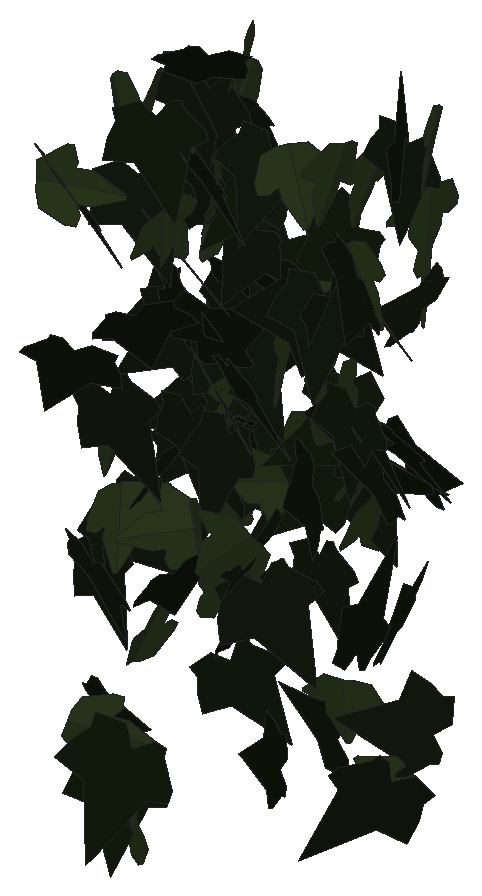
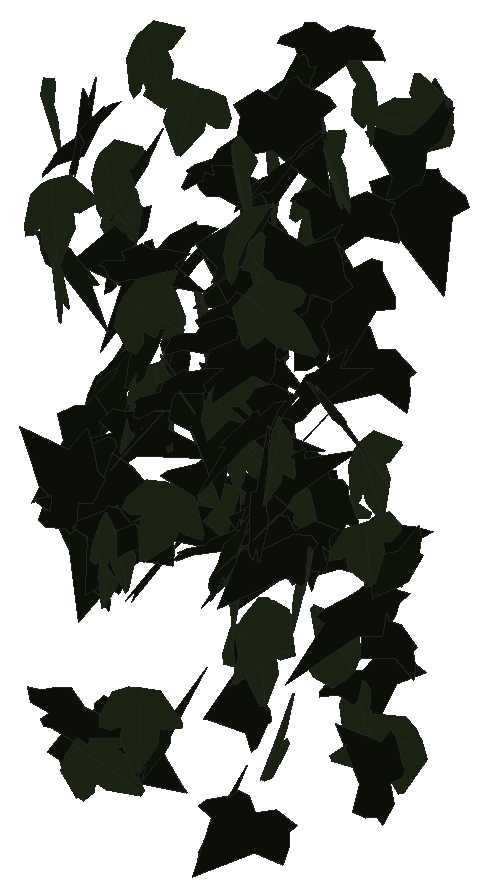
# SketchUp Ruby script. Lengths in inches.
U = 1.inch
M = Sketchup.active_model
def pt(a) = Geom::Point3d.new(a.map { |v| v * U })
def face(e, loops, mat)
  f = e.add_face(loops[0].map { |a| pt(a) })
  loops[1..].each { |l| e.add_face(l.map { |a| pt(a) }).erase! }
  f.material = f.back_material = mat if mat
  f
end
# faces: each face lists its corners as indices into pts; further lists are holes
def faces(e, pts, list, mat = nil) = list.each { |f| face(e, (f[0].is_a?(Array) ? f : [f]).map { |l| l.map { |i| pts[i] } }, mat) }
# xy, xz, yz: faces in a plane at the given z, y or x. An outline is a flat list of corners, or four numbers for a rectangle; further outlines are holes
def ring(l) = l.size == 4 ? [[l[0], l[1]], [l[2], l[1]], [l[2], l[3]], [l[0], l[3]]] : l.each_slice(2).to_a
def flat(e, list, mat, &to3) = list.each { |f| face(e, (f[0].is_a?(Array) ? f : [f]).map { |l| ring(l).map { |u, v| to3.(u, v) } }, mat) }
def xy(e, z, list, mat = nil) = flat(e, list, mat) { |x, y| [x, y, z] }
def xz(e, y, list, mat = nil) = flat(e, list, mat) { |x, z| [x, y, z] }
def yz(e, x, list, mat = nil) = flat(e, list, mat) { |y, z| [x, y, z] }
def lines(e, pts, list) = list.each { |a, b| e.add_line(pt(pts[a]), pt(pts[b])) }
# prism: a flat outline (further loops are holes) pulled along v
def prism(e, loops, v, mat = nil)
  f = face(e, loops, mat); d = Geom::Vector3d.new(v.map { |x| x * U })
  f.pushpull(f.normal.samedirection?(d) ? d.length : -d.length)
end
def box(e, o, s, mat = nil) = prism(e, [[o, [o[0] + s[0], o[1], o[2]], [o[0] + s[0], o[1] + s[1], o[2]], [o[0], o[1] + s[1], o[2]]]], [0, 0, s[2]], mat)
def at(x, y, z, deg = 0) = Geom::Transformation.translation(pt([x, y, z])) * Geom::Transformation.rotation(ORIGIN, Z_AXIS, deg.degrees)
def axes(o, x, y, z) = Geom::Transformation.new([*x, 0, *y, 0, *z, 0, *pt(o).to_a, 1])
def part(name) = M.definitions.add(name)
# library, detail: a bought-in or finely detailed component or shape, given as its bounding box
def library(name, o, s) = part(name).tap { |d| box(d.entities, o, s) }
def detail(e, o, s) = box(e.add_group.entities, o, s)
def put(e, d, t, mat = nil) = e.add_instance(d, t).tap { |i| i.material = mat if mat }
def group(e, t, mat = nil) = e.add_group.tap { |g| g.transformation = t; g.material = mat if mat }.entities
root = M.entities
M.materials.add("efeu1").color = [18, 25, 13]
M.materials.add("efeu2").color = [43, 57, 29]
c1 = part("ivyleaf_9")
p = [[1.54,2.16,1.25],[1.36,2.04,1.19],[-0.21,0.99,0.68],[-0.71,1.11,0.82],[-0.85,0.86,0.67],[-0.8,0.17,0.21],
  [-0.9,-0.01,0.1],[-0.67,-0.16,-0.02],[-0.08,-0.08,-0.05],[-0.03,-0.6,-0.4],[0.65,-0.88,-0.66],[0.83,-0.6,-0.49],
  [1.29,-0.42,-0.43],[1.8125,-0.07,-0.26],[1.21,0.44,0.15]]
faces(c1.entities,p,[[0,1,2,3,4,5,6,7,8,9,10,11,12,13,14]],"efeu1")
c2 = part("ivyleaf_10")
p = [[0,0.5,-0.03],[-0.0625,2.02,-0.43],[-0.19,2.01,-0.46],[-0.54,1.05,-0.29],[-0.52,0.625,-0.18],[-0.83,0.76,-0.28],
  [-1.16,0.64,-0.33],[-1.15,0.33,-0.24],[-0.77,-0.39,0.02],[-0.3,-0.51,0.16],[0.04,-0.48,0.23],[-0.02,2.01,-0.4375],
  [-0.06,2.01,-0.43],[0.04,-0.49,0.23],[0.67,-0.49,0.14],[1.38,0.36,-0.2],[1.375,0.51,-0.24],[0.81,0.65,-0.19],
  [0.62,0.59,-0.15],[0.6,1.09,-0.28],[0.5,1.23,-0.31]]
faces(c2.entities,p,[[0,1,2,3,4,5,6,7,8,9,10],[11,12,0,13,14,15,16,17,18,19,20]],"efeu2")
put(root,c1,axes([616.04,111.68,281.14],[-0.74853,-1.25737,0.03019],[-0.01556,-0.02587,-1.46331],[1.25763,-0.74869,-0.00014]))
put(root,c1,axes([613.32,111.92,296.21],[0.47636,0.77697,-0.89756],[-0.5798,-0.69166,-0.90645],[-1.03592,0.74441,0.0946]))
put(root,c1,axes([613.47,114.57,278.19],[-0.50555,-1.12538,-0.2733],[0.1031,0.25329,-1.23368],[1.15349,-0.51587,-0.00951]))
put(root,c2,axes([614.3125,114.06,276.57],[-0.57352,0.23946,1.0873],[-1.08162,0.17013,-0.60799],[-0.26395,-1.21746,0.1289]))
put(root,c2,axes([610.55,114.28,301.03],[0.01392,0.03971,1.26397],[0.9965,0.77789,-0.03541],[-0.77857,0.99634,-0.02273]))
put(root,c1,axes([610.16,115.37,300.48],[0.78532,-0.97461,0.83994],[0.56308,-0.62446,-1.25104],[1.15686,0.96554,0.03873]))
put(root,c2,axes([618.3,115.15,288.91],[-0.7996,-0.36728,0.91799],[-0.84802,-0.35231,-0.87961],[0.5084,-1.16531,-0.0234]))
put(root,c1,axes([613.84,115.93,304],[-0.46439,-0.92601,-0.72646],[0.44689,0.58375,-1.02977],[1.08882,-0.63454,0.11281]))
put(root,c1,axes([611.9,115.89,292.11],[-0.47109,-0.31019,-1.2433],[1.01351,0.72037,-0.56374],[0.7841,-1.1175,-0.0183]))
put(root,c2,axes([613.66,116.82,300.09],[-0.15625,0.54425,-1.13301],[0.37357,-1.07003,-0.56551],[-1.20015,-0.40392,-0.02852]))
put(root,c1,axes([618.51,115.79,288.34],[-0.65492,1.12217,0.18453],[-0.1139,0.14715,-1.29909],[-1.13153,-0.66432,0.02396]))
put(root,c2,axes([614.82,116.97,287.8125],[-0.50377,0.74151,-0.88779],[0.44004,-0.77267,-0.89506],[-1.06975,-0.66703,0.0499]))
put(root,c1,axes([614.61,116.07,285.93],[0.11253,1.25654,-0.14344],[-0.01769,-0.14242,-1.26156],[-1.26457,0.11381,0.00488]))
put(root,c1,axes([609.91,117.36,284.0625],[0.41715,-1.00323,0.78821],[0.46496,-0.6527,-1.07683],[1.18809,0.60768,0.14467]))
put(root,c1,axes([616,117.21,291.36],[-1.03496,-0.27354,-0.73194],[0.73032,0.09326,-1.06754],[0.27782,-1.26419,0.07962]))
put(root,c1,axes([616.4,117.03,294.24],[0.98176,-0.79741,0.12429],[0.10449,-0.06849,-1.26473],[0.80024,0.98723,0.01266]))
put(root,c1,axes([612.4375,116.55,295.3],[0.60733,1.05679,-0.31651],[-0.14775,-0.28013,-1.21883],[-1.09323,0.62495,-0.01111]))
put(root,c2,axes([610.92,117.5625,303.48],[-0.80775,0.54525,-0.78349],[0.47028,-0.66584,-0.94821],[-0.83066,-0.90718,0.22505]))
put(root,c1,axes([614.23,117.68,301.82],[0.76545,-0.93345,0.51682],[0.33516,-0.39351,-1.20713],[1.01297,0.83556,0.00886]))
put(root,c2,axes([613.7,117.85,286.61],[-0.35213,0.14807,1.18152],[-0.90975,-0.82841,-0.16732],[0.76829,-0.91308,0.3434]))
put(root,c1,axes([614.81,118.05,292.56],[0.53485,-0.74557,0.84956],[0.44755,-0.72337,-0.91658],[1.03794,0.6961,-0.04256]))
put(root,c2,axes([609.78,117.07,277.76],[-0.40708,-0.14289,-1.17115],[1.10499,0.38806,-0.43143],[0.41353,-1.17759,-0.00007]))
put(root,c1,axes([617.44,117.47,285.73],[-0.2332,-0.83855,-1.07303],[0.60266,0.9127,-0.84423],[1.22121,-0.61054,0.21171]))
put(root,c1,axes([619.38,117.71,290.38],[0.18699,-0.00986,-1.45147],[-1.45093,0.03981,-0.18719],[0.04074,1.46292,-0.00468]))
put(root,c2,axes([610.42,118.23,286.4375],[0.5142,1.12279,-0.18676],[-0.07646,-0.17039,-1.23493],[-1.13565,0.51985,-0.00141]))
put(root,c2,axes([612.7,117.86,298.79],[-0.30718,-1.06897,-0.57591],[0.16784,0.55097,-1.1122],[1.20258,-0.34995,0.00812]))
put(root,c2,axes([611.55,118.16,281],[0.21633,-1.16598,0.38725],[-0.00244,0.3928,1.18405],[-1.22861,-0.20608,0.06583]))
put(root,c2,axes([609.99,118.78,289.73],[0.08335,-1.21645,0.30468],[0.11831,-0.29636,-1.21561],[1.24843,0.1093,0.09486]))
put(root,c1,axes([611.03,118.5,299.52],[-0.54887,-0.74019,-0.97444],[0.58866,0.77657,-0.92146],[1.0728,-0.80482,0.00707]))
put(root,c1,axes([608.98,118.81,283.63],[-0.4491,-0.2473,-1.12295],[1.07856,0.32732,-0.50343],[0.39861,-1.16429,0.09699]))
put(root,c1,axes([608.95,118.9,277.32],[0.82916,-0.06966,-0.82887],[0.82688,0.19614,0.81068],[0.09034,-1.15589,0.18751]))
put(root,c1,axes([611.69,118.64,297.75],[1.2303,-0.61089,0.13596],[0.12056,-0.06292,-1.37362],[0.61411,1.23619,-0.00272]))
put(root,c2,axes([619.35,119.29,302.96],[-0.00312,-1.19004,0.44421],[0.14069,-0.4418,-1.1826],[1.26242,0.0463,0.13289]))
put(root,c1,axes([613.51,118.82,293.77],[0.04252,-0.25758,1.32814],[1.32302,-0.26974,-0.09467],[0.28269,1.30115,0.24329]))
put(root,c1,axes([611.59,119.41,294.84],[0.581,-0.096,-1.12494],[1.1199,0.20958,0.56051],[0.1433,-1.24865,0.18057]))
put(root,c1,axes([611.97,118.32,287.95],[-0.12093,1.05167,0.71168],[-0.17347,0.69452,-1.05579],[-1.25794,-0.19688,0.07717]))
put(root,c1,axes([619.43,120.22,297.72],[0.08646,-0.94849,0.9769],[0.16203,-0.96475,-0.95103],[1.35193,0.17628,0.0515]))
put(root,c1,axes([612.3,119.84,289.75],[0.28225,-1.20095,0.23748],[0.10873,-0.21815,-1.23245],[1.21937,0.29744,0.05493]))
put(root,c2,axes([614.05,118.99,300.25],[0.48579,-0.93891,-0.66939],[-0.22818,0.63373,-1.05449],[1.1303,0.53147,0.07482]))
put(root,c2,axes([617.05,119.48,301.9],[1.0239,0.57797,0.36175],[0.2568,0.27772,-1.17056],[-0.63164,1.04981,0.1105]))
put(root,c1,axes([611.2,120.71,292.68],[-0.40424,-0.74245,0.89804],[-0.42027,-0.79367,-0.84533],[1.08678,-0.58309,0.00714]))
put(root,c1,axes([616.95,120.81,295.23],[0.43354,-1.18761,-0.69133],[0.22079,-0.6553,1.26418],[-1.35632,-0.48628,-0.01519]))
put(root,c2,axes([610.24,120.32,302.2],[0.64815,-0.97045,0.48091],[0.28505,-0.38785,-1.16682],[1.04489,0.70778,0.02]))
put(root,c2,axes([616.51,119.78,293.81],[0.75889,-0.96288,-0.33665],[-0.11822,0.33376,-1.22107],[1.01316,0.76017,0.10969]))
put(root,c1,axes([617.68,120.55,296.18],[-0.21093,-1.28899,-0.02219],[0.00089,0.02234,-1.30613],[1.28918,-0.21091,-0.00273]))
put(root,c1,axes([620.05,120.81,289.63],[0.77798,-1.04611,-0.25855],[0.16298,-0.20099,1.30364],[-1.06519,-0.7948,0.01063]))
put(root,c1,axes([618.91,120.75,291.91],[0.04496,-1.1658,0.27314],[0.03402,-0.27198,-1.16644],[1.19689,0.05152,0.02289]))
put(root,c1,axes([615.01,120.89,300.84],[-0.3785,-1.14315,0.21033],[-0.07134,-0.19794,-1.20417],[1.16015,-0.38513,-0.00542]))
put(root,c1,axes([615,120.72,300.02],[-1.16367,-0.36537,0.03234],[-0.03,-0.0124,-1.21968],[0.36556,-1.16406,0.00284]))
put(root,c1,axes([608.95,119.96,284.9],[0.48997,-0.71755,-1.15566],[-0.15903,1.1897,-0.80611],[1.35097,0.40029,0.32424]))
put(root,c1,axes([613.84,121.52,297.06],[-0.30992,-1.05015,0.63585],[0.06055,-0.66807,-1.07386],[1.22615,-0.23244,0.21375]))
put(root,c1,axes([619.67,120.03,282.97],[-0.0094,-0.5434,1.30663],[0.64231,1.16266,0.48815],[-1.26095,0.5963,0.23892]))
put(root,c2,axes([618.86,121,297.92],[-0.9033,0.4476,-0.76053],[0.57777,-0.52265,-0.99384],[-0.66702,-1.05886,0.16906]))
put(root,c1,axes([612.28,120.72,303.93],[0.03022,0.95124,-0.8139],[-0.51569,-0.7324,-0.87513],[-1.14077,0.35628,0.37405]))
put(root,c1,axes([619.75,121.5625,276.79],[-0.02941,0.33739,-1.39931],[-0.14353,-1.39331,-0.33293],[-1.43223,0.1327,0.0621]))
put(root,c2,axes([613.26,121.61,290.61],[0.04173,-1.01204,0.7265],[0.07509,-0.72354,-1.01224],[1.24354,0.07765,0.03675]))
put(root,c1,axes([610.18,120.9,293.02],[-0.97854,0.66687,0.18267],[-0.16146,0.08741,-1.18403],[-0.67232,-0.9916,0.01848]))
put(root,c1,axes([611.61,122.1875,289.39],[0.18406,-0.85984,-1.05865],[0.21611,-1.03636,0.87931],[-1.34661,-0.28384,-0.00358]))
put(root,c1,axes([611.125,121.61,302.4375],[0.17635,-1.26022,-0.02444],[-0.00533,0.02393,-1.2725],[1.26044,0.17642,-0.00196]))
put(root,c1,axes([611.61,121.71,301.8],[0.05761,-1.28584,-0.10032],[-0.00409,0.10024,-1.28713],[1.28974,0.05776,0.0004]))
put(root,c1,axes([617.51,122.08,290.12],[0.78541,-0.95257,-0.33443],[0.22928,-0.24434,1.23443],[-0.98318,-0.81793,0.02072]))
put(root,c1,axes([617.8125,120.84,296.02],[0.42516,-0.73412,-1.04501],[-0.52003,0.90644,-0.84835],[1.16643,0.67171,0.00268]))
put(root,c1,axes([618.21,121.57,296.57],[0.9033,-0.72708,0.40505],[0.30799,-0.26333,-1.15951],[0.77321,0.9543,-0.01134]))
put(root,c1,axes([613.14,121.29,292.42],[-0.33448,-0.70921,-1.06674],[0.55914,0.9111,-0.78106],[1.15251,-0.64785,0.06934]))
put(root,c1,axes([616.65,121.6875,284.76],[0.49193,-1.17285,-0.11904],[-0.03254,0.11542,-1.27175],[1.17842,0.49279,0.01457]))
put(root,c1,axes([613.51,121.35,290.8],[-0.58062,0.49092,0.97923],[-1.00135,0.21142,-0.69972],[-0.44406,-1.11862,0.2975]))
put(root,c1,axes([610.59,121.25,297.37],[-0.37749,-0.04199,1.26437],[1.22567,-0.33884,0.35469],[0.31323,1.27527,0.13587]))
put(root,c2,axes([617.45,121.19,291.26],[-0.94798,0.22178,0.68669],[-0.68901,0.05878,-0.97016],[-0.21448,-1.16908,0.08149]))
put(root,c2,axes([614.67,121.36,287.36],[0.45816,-0.10124,-1.08289],[-1.05072,0.26228,-0.46907],[0.28089,1.1462,0.01169]))
put(root,c2,axes([617.05,121.62,295.39],[1.15489,-0.21825,0.33949],[0.34635,0.00766,-1.1733],[0.2072,1.20373,0.06902]))
put(root,c2,axes([612.24,121.67,297.3125],[1.02159,-0.59653,-0.373],[-0.30013,0.22528,-1.18228],[0.63631,1.06397,0.0412]))
put(root,c1,axes([618.24,121.91,290.87],[0.85256,-0.87466,0.2312],[0.15542,-0.17136,-1.22141],[0.89126,0.86658,-0.00817]))
put(root,c1,axes([612.41,121.17,287.26],[1.03182,-0.26269,-0.64957],[-0.47676,0.58411,-0.99354],[0.51347,1.07024,0.38281]))
put(root,c2,axes([612.46,121.84,283.1],[-1.09832,-0.17416,0.35895],[-0.35124,-0.0766,-1.11187],[0.18924,-1.15295,0.01965]))
put(root,c1,axes([616.57,122.57,277.14],[0.49366,-1.17901,0.11255],[-0.02265,0.11251,1.27799],[-1.18416,-0.49367,0.02248]))
put(root,c2,axes([619.3,122.63,276.375],[-0.42151,-0.57488,0.96177],[-0.52051,-0.8095,-0.71199],[0.99225,-0.66886,0.03507]))
put(root,c1,axes([613.74,122.95,274.75],[-0.22734,0.02277,1.13693],[-0.28328,-1.12401,-0.03413],[1.10131,-0.28442,0.22592]))
put(root,c1,axes([612.72,121.71,295.12],[1.2042,0.31475,-0.16015],[-0.15402,-0.04406,-1.24465],[-0.3178,1.214,-0.00365]))
put(root,c1,axes([620.47,121.15,283.49],[-0.18276,0.95519,1.06688],[-0.15762,1.05558,-0.97208],[-1.4233,-0.23955,-0.02934]))
put(root,c2,axes([613.18,122.86,292.55],[0.03604,-1.07618,0.63458],[-0.00304,-0.63492,-1.07658],[1.24934,0.02951,-0.02093]))
put(root,c1,axes([615.92,123.0625,287.18],[-1.04009,-0.59,0.39192],[-0.34341,-0.18893,-1.19577],[0.61949,-1.09531,-0.00485]))
put(root,c1,axes([617.55,123.125,290.02],[-1.08039,-0.45228,0.729],[-0.67138,-0.28408,-1.17123],[0.53409,-1.272,0.00237]))
put(root,c1,axes([610.66,122.02,287.95],[-0.00672,-0.69302,-1.08896],[0.03147,1.08856,-0.69296],[1.29039,-0.03016,0.01123]))
put(root,c2,axes([617.3,121.97,291.63],[0.1902,-0.93641,-0.81977],[0.10181,0.83821,-0.93386],[1.24037,0.07479,0.20235]))
put(root,c1,axes([612.59,121.53,280.65],[0.15764,0.44256,1.24519],[0.34735,1.19605,-0.46907],[-1.27503,0.38055,0.02617]))
put(root,c2,axes([617.01,122.64,279.1875],[-1.097,-0.40835,0.09557],[-0.08449,-0.04696,-1.17044],[0.41078,-1.10015,0.01448]))
put(root,c1,axes([616.75,123.47,297.3],[-1.00828,-0.64966,0.29713],[-0.2128,-0.21748,-1.19766],[0.68195,-1.0284,0.06557]))
put(root,c2,axes([609.8,122.43,287.1875],[-0.82464,0.76915,0.3218],[-0.23719,0.21749,-1.12766],[-0.79931,-0.85807,0.00263]))
put(root,c1,axes([616.09,123.52,290.69],[0.16329,-1.15416,0.38697],[0.10739,-0.37526,-1.16454],[1.21256,0.18866,0.05102]))
put(root,c1,axes([619.07,123.55,301.41],[0.05009,-1.23206,0.26626],[-0.03011,-0.26756,-1.23243],[1.26014,0.04258,-0.04003]))
put(root,c1,axes([610.77,122.16,287.9],[1.00385,0.61352,0.20599],[0.14342,0.15982,-1.17493],[-0.63109,1.01223,0.06066]))
put(root,c1,axes([613.57,123.57,295.61],[-0.61101,-1.04199,0.06481],[0.06964,-0.11561,-1.20211],[1.04168,-0.60346,0.11838]))
put(root,c1,axes([613.05,123.73,287.47],[-0.57496,-1.04397,0.24353],[0.15409,-0.35396,-1.15357],[1.06086,-0.51439,0.29954]))
put(root,c2,axes([617.77,123.33,300.55],[0.12509,-1.17731,0.40735],[0.09946,-0.39866,-1.18272],[1.24182,0.15052,0.0537]))
put(root,c1,axes([620.49,122.49,295.85],[-0.58717,0.96709,0.40811],[-0.37691,0.24218,-1.11618],[-0.97967,-0.6728,0.18483]))
put(root,c1,axes([615.15,123.09,293.18],[-1.08795,0.44277,-0.26856],[0.25092,-0.09588,-1.17458],[-0.453,-1.11649,-0.00563]))
put(root,c1,axes([616.17,123.71,293.39],[-0.47843,-0.05091,1.13101],[0.05547,-1.22742,-0.03179],[1.13079,0.03867,0.48008]))
put(root,c1,axes([619.5,122.6875,300.66],[0.04651,-0.67229,1.10508],[0.14571,1.10148,0.66397],[-1.28528,0.10054,0.11527]))
put(root,c2,axes([610.78,122.52,291.87],[0.14696,-0.72313,-0.979],[-0.126,0.97177,-0.7367],[1.21057,0.18893,0.04217]))
put(root,c2,axes([612.4,122.71,286.38],[-0.40548,0.94822,0.55284],[-0.44459,0.39695,-1.00694],[-1.00354,-0.55899,0.22273]))
put(root,c1,axes([620.09,123.48,278.15],[-0.78892,0.19747,0.95868],[-0.9543,0.1186,-0.80975],[-0.21763,-1.23588,0.07547]))
put(root,c2,axes([615.85,124.16,296.13],[-0.22494,-0.75898,0.99529],[0.01683,-1.01298,-0.76866],[1.25155,-0.12279,0.18922]))
put(root,c2,axes([611.0625,122.91,284.85],[-0.21967,-0.9108,-0.79876],[0.27563,0.75292,-0.93433],[1.17966,-0.34552,0.06956]))
put(root,c1,axes([613.62,122.89,292.6875],[-0.18387,1.24997,0.05276],[-0.01554,0.05104,-1.2634],[-1.25099,-0.18436,0.00794]))
put(root,c1,axes([611.84,124.37,287.08],[-0.12793,-0.43461,1.20596],[0.18294,-1.20573,-0.41512],[1.26876,0.13003,0.18146]))
put(root,c2,axes([611.86,123.5,302.95],[0.55248,-1.11838,-0.16451],[-0.03928,0.164,-1.24685],[1.12973,0.55263,0.0371]))
put(root,c2,axes([619.97,123.94,302.5],[0.76211,-0.91244,0.40984],[0.29454,-0.2877,-1.1882],[0.95591,0.8161,0.03936]))
put(root,c1,axes([618.36,123.26,289.66],[1.18606,-0.10363,-0.0657],[-0.06498,0.01105,-1.19056],[0.10408,1.18782,0.00534]))
put(root,c2,axes([617.375,123.59,286.26],[-0.02904,-1.13651,-0.47139],[0.06541,0.46942,-1.13581],[1.22865,-0.05186,0.04933]))
put(root,c2,axes([609.84,124.25,280.12],[-0.53137,0.89456,0.65066],[0.31712,-0.56835,1.04037],[1.05973,0.61863,0.01493]))
put(root,c1,axes([610.97,124.23,300.4375],[0.67751,-0.9239,0.43684],[0.38317,-0.25623,-1.1362],[0.94741,0.76432,0.14713]))
put(root,c2,axes([614.75,123.86,288.61],[-1.11479,-0.29345,-0.3124],[0.3142,0.03256,-1.15182],[0.29152,-1.15728,0.04681]))
put(root,c1,axes([610.1,124.68,289.18],[-0.05431,0.44264,1.33266],[-0.14423,-1.32836,0.43534],[1.39682,-0.11995,0.09676]))
put(root,c2,axes([610.82,124.74,300.92],[-0.02268,-0.9765,0.74349],[0.36447,-0.71543,-0.92853],[1.17196,0.20359,0.30315]))
put(root,c1,axes([616.32,123.96,287.43],[0.77833,-0.17336,0.99952],[0.96786,-0.25047,-0.79712],[0.30388,1.24181,-0.02124]))
put(root,c2,axes([619.3125,124.32,296.64],[0.85503,-0.82679,0.25427],[0.30571,-0.04562,-1.17634],[0.80918,0.89087,0.17574]))
put(root,c1,axes([614.09,124.93,293.69],[-0.5805,-1.02823,0.31517],[-0.12521,-0.2911,-1.18032],[1.06813,-0.59294,0.03293]))
put(root,c1,axes([610.86,123.78,293.17],[0.56315,-0.72783,-0.80416],[-0.28944,0.77239,-0.90177],[1.0453,0.60599,0.18354]))
put(root,c1,axes([616.3125,124.04,287.18],[-0.37368,-0.70522,-0.99888],[0.42377,0.90505,-0.79751],[1.14695,-0.56416,-0.03077]))
put(root,c2,axes([619.5,124.27,299.18],[-0.3119,-1.20336,0.01364],[0.09497,-0.03865,-1.23896],[1.19968,-0.30979,0.10163]))
put(root,c2,axes([610.32,124.2,298.125],[0.68811,0.32757,-0.9884],[-1.03154,0.05294,-0.70061],[-0.14195,1.20317,0.29993]))
put(root,c1,axes([610.9,123.9375,277.53],[-0.26868,-0.43023,-1.11387],[0.53512,0.97727,-0.50655],[1.06745,-0.5982,-0.02643]))
put(root,c1,axes([610.19,124.98,289.09],[-0.02401,-1.1326,0.44618],[0.15102,-0.44559,-1.12298],[1.20792,0.0332,0.14927]))
put(root,c2,axes([616.67,124.36,287.16],[0.04492,-1.17309,0.03024],[-0.0109,-0.03068,-1.17388],[1.17343,0.04462,-0.01206]))
put(root,c1,axes([618.16,124.71,287.9],[0.28611,-0.38955,1.27046],[0.88399,-0.91452,-0.47949],[0.99216,0.92714,0.06084]))
